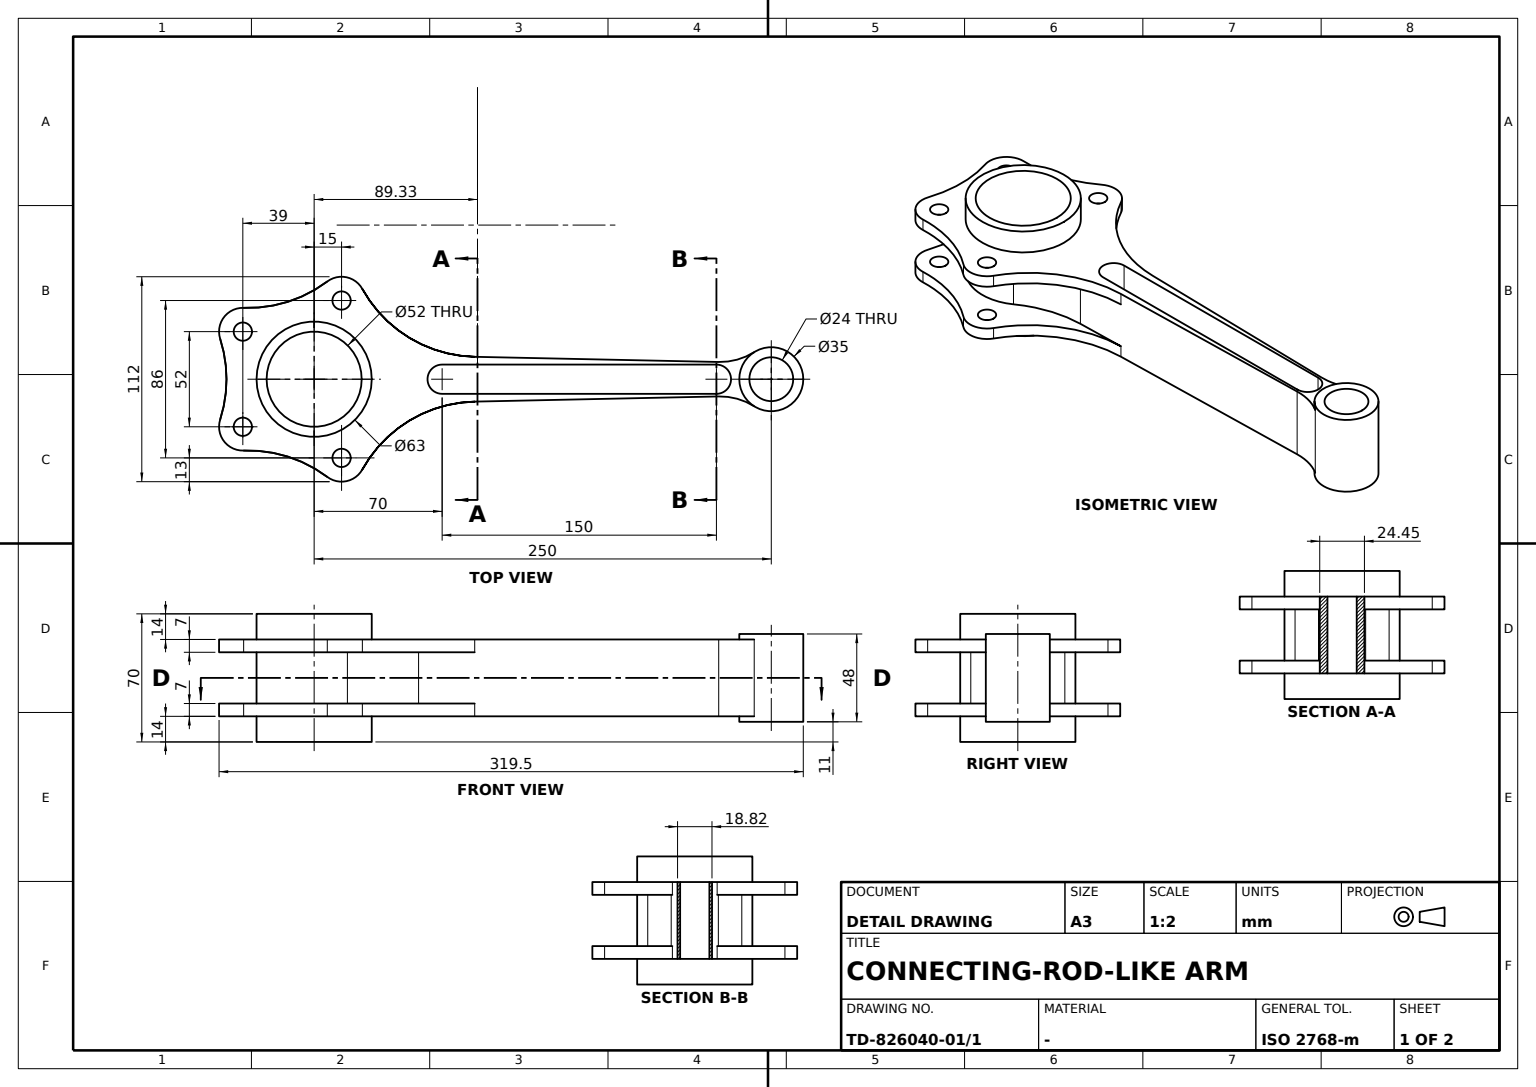
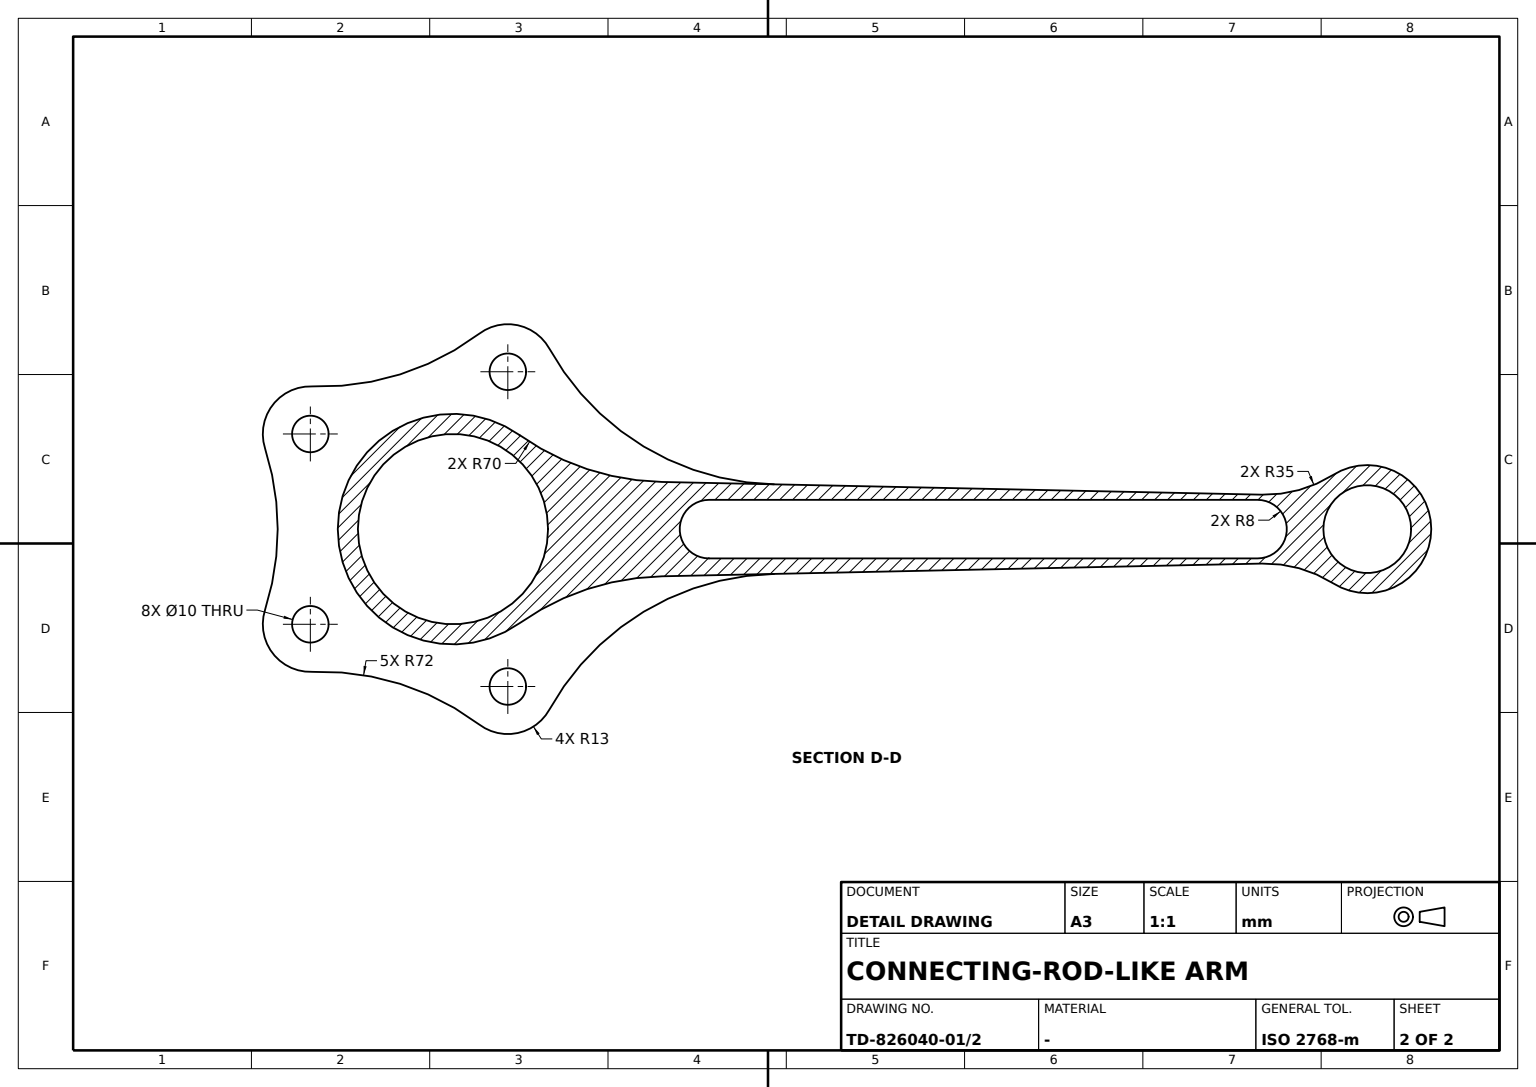
solid
v1 (7.189691,-53.392261,-14)
v2 (-38.551485,-38.992261,-14)
e1 v1 v2 CIRCLE(AX(P(-36.067402,-110.949396,-14),D(0,0,1),D(1,0,0)),72)
v3 (-38.551485,-38.992261,-21)
e2 v2 v3 LINE
v4 (7.189691,-53.392261,-21)
e3 v4 v3 CIRCLE(AX(P(-36.067402,-110.949396,-21),D(0,0,1),D(1,0,0)),72)
e4 v1 v4 LINE
face CYL(AX(P(-36.067402,-110.949396,17.5),D(0,0,1),D(1,0,0)),72) rev [e1 e2 -e3 -e4]
v5 (-38.551485,38.992261,-14)
v6 (7.189691,53.392261,-14)
e5 v5 v6 CIRCLE(AX(P(-36.067402,110.949396,-14),D(0,0,1),D(1,0,0)),72)
v7 (7.189691,53.392261,-21)
e6 v6 v7 LINE
v8 (-38.551485,38.992261,-21)
e7 v8 v7 CIRCLE(AX(P(-36.067402,110.949396,-21),D(0,0,1),D(1,0,0)),72)
e8 v5 v8 LINE
face CYL(AX(P(-36.067402,110.949396,17.5),D(0,0,1),D(1,0,0)),72) rev [e5 e6 -e7 -e8]
v9 (262,0,24)
e9 v9 v9 CIRCLE(AX(P(250,0,24),D(0,0,1),D(1,0,0)),12)
v10 (262,0,-24)
e10 v10 v10 CIRCLE(AX(P(250,0,-24),D(0,0,1),D(1,0,0)),12)
face CYL(AX(P(250,0,0),D(0,0,1),D(1,0,0)),12) rev [e9] [-e10]
v11 (31.5,0,-21)
e11 v11 v11 CIRCLE(AX(P(0,0,-21),D(0,0,1),D(1,0,0)),31.5)
v12 (31.5,0,-35)
e12 v12 v12 CIRCLE(AX(P(0,0,-35),D(0,0,1),D(1,0,0)),31.5)
face CYL(AX(P(0,0,0),D(0,0,1),D(1,0,0)),31.5) [-e11] [e12]
v13 (-51.376901,-22.023529,21)
v14 (-38.551485,-38.992261,21)
e13 v13 v14 CIRCLE(AX(P(-39,-26,21),D(0,0,1),D(1,0,0)),13)
v15 (-51.376901,-22.023529,14)
e14 v13 v15 LINE
v16 (-38.551485,-38.992261,14)
e15 v15 v16 CIRCLE(AX(P(-39,-26,14),D(0,0,1),D(1,0,0)),13)
e16 v14 v16 LINE
face CYL(AX(P(-39,-26,17.5),D(0,0,1),D(1,0,0)),13) [-e13 e14 e15 -e16]
v17 (57.116555,12.890905,-14)
v18 (57.116555,12.890905,14)
e17 v17 v18 LINE
v19 (87.808379,12.240359,14)
e18 v18 v19 LINE
v20 (87.808379,12.240359,21)
e19 v20 v19 LINE
v21 (221.248896,9.411947,21)
e20 v20 v21 LINE
v22 (221.248896,9.411947,-21)
e21 v22 v21 LINE
v23 (87.808379,12.240359,-21)
e22 v23 v22 LINE
v24 (87.808379,12.240359,-14)
e23 v24 v23 LINE
e24 v17 v24 LINE
face PLANE(AX(P(57.116555,12.890905,0),D(-0.02119129,-0.999775439,0),D(0.999775439,-0.02119129,0))) rev [e17 e18 -e19 e20 -e21 -e22 -e23 -e24]
v25 (-34,26,21)
e25 v25 v25 CIRCLE(AX(P(-39,26,21),D(0,0,1),D(1,0,0)),5)
v26 (-34,26,14)
e26 v26 v26 CIRCLE(AX(P(-39,26,14),D(0,0,1),D(1,0,0)),5)
face CYL(AX(P(-39,26,17.5),D(0,0,1),D(1,0,0)),5) rev [e25] [-e26]
v27 (26.368753,49.304876,21)
e27 v27 v20 CIRCLE(AX(P(89.334152,84.224191,21),D(0,0,1),D(1,0,0)),72)
v28 (26.368753,49.304876,14)
e28 v28 v19 CIRCLE(AX(P(89.334152,84.224191,14),D(0,0,1),D(1,0,0)),72)
e29 v27 v28 LINE
face CYL(AX(P(89.334152,84.224191,17.5),D(0,0,1),D(1,0,0)),72) rev [e27 e19 -e28 -e29]
v29 (20,43,-21)
e30 v29 v29 CIRCLE(AX(P(15,43,-21),D(0,0,1),D(1,0,0)),5)
v30 (240.66353,14.801363,-21)
e31 v22 v30 CIRCLE(AX(P(221.990591,44.404088,-21),D(0,0,1),D(1,0,0)),35)
v31 (240.66353,-14.801363,-21)
e32 v30 v31 CIRCLE(AX(P(250,0,-21),D(0,0,1),D(1,0,0)),17.5)
v32 (221.248896,-9.411947,-21)
e33 v31 v32 CIRCLE(AX(P(221.990591,-44.404088,-21),D(0,0,1),D(1,0,0)),35)
v33 (87.808379,-12.240359,-21)
e34 v33 v32 LINE
v34 (26.368753,-49.304876,-21)
e35 v33 v34 CIRCLE(AX(P(89.334152,-84.224191,-21),D(0,0,1),D(1,0,0)),72)
e36 v4 v34 CIRCLE(AX(P(15,-43,-21),D(0,0,1),D(1,0,0)),13)
v35 (-51.376901,-22.023529,-21)
e37 v35 v3 CIRCLE(AX(P(-39,-26,-21),D(0,0,1),D(1,0,0)),13)
v36 (-51.376901,22.023529,-21)
e38 v35 v36 CIRCLE(AX(P(-119.925892,0,-21),D(0,0,1),D(1,0,0)),72)
e39 v8 v36 CIRCLE(AX(P(-39,26,-21),D(0,0,1),D(1,0,0)),13)
v37 (26.368753,49.304876,-21)
e40 v37 v7 CIRCLE(AX(P(15,43,-21),D(0,0,1),D(1,0,0)),13)
e41 v37 v23 CIRCLE(AX(P(89.334152,84.224191,-21),D(0,0,1),D(1,0,0)),72)
v38 (-34,-26,-21)
e42 v38 v38 CIRCLE(AX(P(-39,-26,-21),D(0,0,1),D(1,0,0)),5)
v39 (20,-43,-21)
e43 v39 v39 CIRCLE(AX(P(15,-43,-21),D(0,0,1),D(1,0,0)),5)
v40 (-34,26,-21)
e44 v40 v40 CIRCLE(AX(P(-39,26,-21),D(0,0,1),D(1,0,0)),5)
v41 (70,8,-21)
v42 (220,8,-21)
e45 v41 v42 LINE
v43 (70,-8,-21)
e46 v41 v43 CIRCLE(AX(P(70,0,-21),D(0,0,1),D(1,0,0)),8)
v44 (220,-8,-21)
e47 v44 v43 LINE
e48 v44 v42 CIRCLE(AX(P(220,0,-21),D(0,0,1),D(1,0,0)),8)
face PLANE(AX(P(0,0,-21),D(0,0,1),D(1,0,0))) rev [e30] [e22 e31 e32 e33 -e34 e35 -e36 e3 -e37 e38 -e39 e7 -e40 e41] [e42] [e43] [e11] [e44] [-e45 e46 -e47 e48]
v45 (7.189691,-53.392261,14)
v46 (26.368753,-49.304876,14)
e49 v45 v46 CIRCLE(AX(P(15,-43,14),D(0,0,1),D(1,0,0)),13)
v47 (26.368753,-49.304876,21)
e50 v47 v46 LINE
v48 (7.189691,-53.392261,21)
e51 v48 v47 CIRCLE(AX(P(15,-43,21),D(0,0,1),D(1,0,0)),13)
e52 v48 v45 LINE
face CYL(AX(P(15,-43,17.5),D(0,0,1),D(1,0,0)),13) [e49 -e50 -e51 e52]
v49 (87.808379,-12.240359,-14)
e53 v33 v49 LINE
v50 (26.368753,-49.304876,-14)
e54 v49 v50 CIRCLE(AX(P(89.334152,-84.224191,-14),D(0,0,1),D(1,0,0)),72)
e55 v50 v34 LINE
face CYL(AX(P(89.334152,-84.224191,17.5),D(0,0,1),D(1,0,0)),72) rev [-e35 e53 e54 e55]
v51 (221.248896,-9.411947,21)
e56 v32 v51 LINE
v52 (87.808379,-12.240359,21)
e57 v52 v51 LINE
v53 (87.808379,-12.240359,14)
e58 v53 v52 LINE
v54 (57.116555,-12.890905,14)
e59 v54 v53 LINE
v55 (57.116555,-12.890905,-14)
e60 v55 v54 LINE
e61 v55 v49 LINE
face PLANE(AX(P(57.116555,-12.890905,0),D(0.02119129,-0.999775439,0),D(0.999775439,0.02119129,0))) [-e53 e34 e56 -e57 -e58 -e59 -e60 e61]
v56 (26.368753,49.304876,-14)
e62 v56 v6 CIRCLE(AX(P(15,43,-14),D(0,0,1),D(1,0,0)),13)
e63 v56 v37 LINE
face CYL(AX(P(15,43,17.5),D(0,0,1),D(1,0,0)),13) [e40 -e6 -e62 e63]
v57 (26,0,35)
e64 v57 v57 CIRCLE(AX(P(0,0,35),D(0,0,1),D(1,0,0)),26)
v58 (31.5,0,35)
e65 v58 v58 CIRCLE(AX(P(0,0,35),D(0,0,1),D(1,0,0)),31.5)
face PLANE(AX(P(0,0,35),D(0,0,1),D(1,0,0))) [-e64] [e65]
v59 (20,43,-14)
e66 v59 v59 CIRCLE(AX(P(15,43,-14),D(0,0,1),D(1,0,0)),5)
face CYL(AX(P(15,43,17.5),D(0,0,1),D(1,0,0)),5) rev [e66] [-e30]
v60 (-51.376901,22.023529,-14)
e67 v5 v60 CIRCLE(AX(P(-39,26,-14),D(0,0,1),D(1,0,0)),13)
e68 v60 v36 LINE
face CYL(AX(P(-39,26,17.5),D(0,0,1),D(1,0,0)),13) [-e67 e8 e39 -e68]
v61 (31.5,0,21)
e69 v61 v61 CIRCLE(AX(P(0,0,21),D(0,0,1),D(1,0,0)),31.5)
face CYL(AX(P(0,0,0),D(0,0,1),D(1,0,0)),31.5) [-e65] [e69]
v62 (18.18619,25.719885,14)
v63 (18.18619,-25.719885,14)
e70 v62 v63 CIRCLE(AX(P(0,0,14),D(0,0,1),D(1,0,0)),31.5)
v64 (18.18619,25.719885,-14)
e71 v64 v62 LINE
v65 (18.18619,-25.719885,-14)
e72 v64 v65 CIRCLE(AX(P(0,0,-14),D(0,0,1),D(1,0,0)),31.5)
e73 v65 v63 LINE
face CYL(AX(P(0,0,0),D(0,0,1),D(1,0,0)),31.5) [-e70 -e71 e72 e73]
v66 (267.5,0,-24)
e74 v66 v66 CIRCLE(AX(P(250,0,-24),D(0,0,1),D(1,0,0)),17.5)
face PLANE(AX(P(0,0,-24),D(0,0,1),D(1,0,0))) rev [-e74] [e10]
v67 (267.5,0,24)
e75 v67 v67 CIRCLE(AX(P(250,0,24),D(0,0,1),D(1,0,0)),17.5)
face PLANE(AX(P(0,0,24),D(0,0,1),D(1,0,0))) [-e9] [e75]
v68 (20,-43,21)
e76 v68 v68 CIRCLE(AX(P(15,-43,21),D(0,0,1),D(1,0,0)),5)
v69 (20,-43,14)
e77 v69 v69 CIRCLE(AX(P(15,-43,14),D(0,0,1),D(1,0,0)),5)
face CYL(AX(P(15,-43,17.5),D(0,0,1),D(1,0,0)),5) rev [e76] [-e77]
v70 (70,8,21)
v71 (220,8,21)
e78 v70 v71 LINE
e79 v70 v41 LINE
e80 v42 v71 LINE
face PLANE(AX(P(70,8,0),D(0,-1,0),D(1,0,0))) [-e78 e79 e45 e80]
v72 (-34,-26,14)
e81 v72 v72 CIRCLE(AX(P(-39,-26,14),D(0,0,1),D(1,0,0)),5)
v73 (20,43,14)
e82 v73 v73 CIRCLE(AX(P(15,43,14),D(0,0,1),D(1,0,0)),5)
e83 v62 v18 CIRCLE(AX(P(58.599946,82.875185,14),D(0,0,1),D(1,0,0)),70)
e84 v54 v63 CIRCLE(AX(P(58.599946,-82.875185,14),D(0,0,1),D(1,0,0)),70)
e85 v53 v46 CIRCLE(AX(P(89.334152,-84.224191,14),D(0,0,1),D(1,0,0)),72)
e86 v45 v16 CIRCLE(AX(P(-36.067402,-110.949396,14),D(0,0,1),D(1,0,0)),72)
v74 (-51.376901,22.023529,14)
e87 v15 v74 CIRCLE(AX(P(-119.925892,0,14),D(0,0,1),D(1,0,0)),72)
v75 (-38.551485,38.992261,14)
e88 v75 v74 CIRCLE(AX(P(-39,26,14),D(0,0,1),D(1,0,0)),13)
v76 (7.189691,53.392261,14)
e89 v75 v76 CIRCLE(AX(P(-36.067402,110.949396,14),D(0,0,1),D(1,0,0)),72)
e90 v28 v76 CIRCLE(AX(P(15,43,14),D(0,0,1),D(1,0,0)),13)
face PLANE(AX(P(0,0,14),D(0,0,1),D(1,0,0))) rev [e77] [e81] [e82] [e26] [-e18 -e83 e70 -e84 e59 e85 -e49 e86 -e15 e87 -e88 e89 -e90 e28]
v77 (220,-8,21)
e91 v77 v71 CIRCLE(AX(P(220,0,21),D(0,0,1),D(1,0,0)),8)
e92 v44 v77 LINE
face CYL(AX(P(220,0,0),D(0,0,1),D(1,0,0)),8) rev [e91 -e80 -e48 e92]
v78 (-34,-26,-14)
e93 v78 v78 CIRCLE(AX(P(-39,-26,-14),D(0,0,1),D(1,0,0)),5)
face CYL(AX(P(-39,-26,17.5),D(0,0,1),D(1,0,0)),5) rev [e93] [-e42]
e94 v1 v50 CIRCLE(AX(P(15,-43,-14),D(0,0,1),D(1,0,0)),13)
face CYL(AX(P(15,-43,17.5),D(0,0,1),D(1,0,0)),13) [e36 -e55 -e94 e4]
e95 v48 v14 CIRCLE(AX(P(-36.067402,-110.949396,21),D(0,0,1),D(1,0,0)),72)
face CYL(AX(P(-36.067402,-110.949396,17.5),D(0,0,1),D(1,0,0)),72) rev [e95 e16 -e86 -e52]
v79 (20,43,21)
e96 v79 v79 CIRCLE(AX(P(15,43,21),D(0,0,1),D(1,0,0)),5)
face CYL(AX(P(15,43,17.5),D(0,0,1),D(1,0,0)),5) rev [e96] [-e82]
v80 (-34,26,-14)
e97 v80 v80 CIRCLE(AX(P(-39,26,-14),D(0,0,1),D(1,0,0)),5)
e98 v64 v17 CIRCLE(AX(P(58.599946,82.875185,-14),D(0,0,1),D(1,0,0)),70)
e99 v56 v24 CIRCLE(AX(P(89.334152,84.224191,-14),D(0,0,1),D(1,0,0)),72)
v81 (-51.376901,-22.023529,-14)
e100 v81 v60 CIRCLE(AX(P(-119.925892,0,-14),D(0,0,1),D(1,0,0)),72)
e101 v81 v2 CIRCLE(AX(P(-39,-26,-14),D(0,0,1),D(1,0,0)),13)
e102 v55 v65 CIRCLE(AX(P(58.599946,-82.875185,-14),D(0,0,1),D(1,0,0)),70)
v82 (20,-43,-14)
e103 v82 v82 CIRCLE(AX(P(15,-43,-14),D(0,0,1),D(1,0,0)),5)
face PLANE(AX(P(0,0,-14),D(0,0,1),D(1,0,0))) [-e66] [-e93] [-e97] [-e72 e98 e24 -e99 e62 -e5 e67 -e100 e101 -e1 e94 -e54 -e61 e102] [-e103]
v83 (26,0,-35)
e104 v83 v83 CIRCLE(AX(P(0,0,-35),D(0,0,1),D(1,0,0)),26)
face CYL(AX(P(0,0,0),D(0,0,1),D(1,0,0)),26) rev [-e104] [e64]
v84 (70,-8,21)
e105 v70 v84 CIRCLE(AX(P(70,0,21),D(0,0,1),D(1,0,0)),8)
e106 v84 v43 LINE
face CYL(AX(P(70,0,0),D(0,0,1),D(1,0,0)),8) rev [-e79 e105 e106 -e46]
v85 (240.66353,-14.801363,21)
e107 v31 v85 LINE
v86 (240.66353,14.801363,21)
e108 v30 v86 LINE
e109 v86 v85 CIRCLE(AX(P(250,0,21),D(0,0,1),D(1,0,0)),17.5)
face CYL(AX(P(250,0,0),D(0,0,1),D(1,0,0)),17.5) [-e107 -e32 e108 e109] [e74] [-e75]
v87 (-51.376901,22.023529,21)
e110 v13 v87 CIRCLE(AX(P(-119.925892,0,21),D(0,0,1),D(1,0,0)),72)
e111 v87 v74 LINE
face CYL(AX(P(-119.925892,0,17.5),D(0,0,1),D(1,0,0)),72) rev [-e14 e110 e111 -e87]
face CYL(AX(P(58.599946,82.875185,0),D(0,0,1),D(1,0,0)),70) rev [-e17 -e98 e71 e83]
e112 v52 v47 CIRCLE(AX(P(89.334152,-84.224191,21),D(0,0,1),D(1,0,0)),72)
face CYL(AX(P(89.334152,-84.224191,17.5),D(0,0,1),D(1,0,0)),72) rev [-e85 e58 e112 e50]
face CYL(AX(P(-39,26,17.5),D(0,0,1),D(1,0,0)),5) rev [e97] [-e44]
face CYL(AX(P(58.599946,-82.875185,0),D(0,0,1),D(1,0,0)),70) rev [e60 e84 -e73 -e102]
v88 (-38.551485,38.992261,21)
v89 (7.189691,53.392261,21)
e113 v88 v89 CIRCLE(AX(P(-36.067402,110.949396,21),D(0,0,1),D(1,0,0)),72)
e114 v89 v76 LINE
e115 v88 v75 LINE
face CYL(AX(P(-36.067402,110.949396,17.5),D(0,0,1),D(1,0,0)),72) rev [e113 e114 -e89 -e115]
e116 v21 v86 CIRCLE(AX(P(221.990591,44.404088,21),D(0,0,1),D(1,0,0)),35)
face CYL(AX(P(221.990591,44.404088,0),D(0,0,1),D(1,0,0)),35) rev [e21 e116 -e108 -e31]
e117 v81 v35 LINE
face CYL(AX(P(-39,-26,17.5),D(0,0,1),D(1,0,0)),13) [-e101 e117 e37 -e2]
e118 v77 v84 LINE
face PLANE(AX(P(220,-8,0),D(0,1,0),D(-1,0,0))) [-e92 e47 -e106 -e118]
face CYL(AX(P(-119.925892,0,17.5),D(0,0,1),D(1,0,0)),72) rev [e68 -e38 -e117 e100]
face PLANE(AX(P(0,0,-35),D(0,0,1),D(1,0,0))) rev [e104] [-e12]
e119 v88 v87 CIRCLE(AX(P(-39,26,21),D(0,0,1),D(1,0,0)),13)
face CYL(AX(P(-39,26,17.5),D(0,0,1),D(1,0,0)),13) [e115 e88 -e111 -e119]
e120 v27 v89 CIRCLE(AX(P(15,43,21),D(0,0,1),D(1,0,0)),13)
face CYL(AX(P(15,43,17.5),D(0,0,1),D(1,0,0)),13) [-e114 -e120 e29 e90]
e121 v85 v51 CIRCLE(AX(P(221.990591,-44.404088,21),D(0,0,1),D(1,0,0)),35)
face CYL(AX(P(221.990591,-44.404088,0),D(0,0,1),D(1,0,0)),35) rev [e107 e121 -e56 -e33]
v90 (-34,-26,21)
e122 v90 v90 CIRCLE(AX(P(-39,-26,21),D(0,0,1),D(1,0,0)),5)
face PLANE(AX(P(0,0,21),D(0,0,1),D(1,0,0))) [-e122] [-e96] [-e76] [-e91 e118 -e105 e78] [-e25] [-e95 e51 -e112 e57 -e121 -e109 -e116 -e20 -e27 e120 -e113 e119 -e110 e13] [-e69]
face CYL(AX(P(15,-43,17.5),D(0,0,1),D(1,0,0)),5) rev [-e43] [e103]
face CYL(AX(P(-39,-26,17.5),D(0,0,1),D(1,0,0)),5) rev [e122] [-e81]
face CYL(AX(P(89.334152,84.224191,17.5),D(0,0,1),D(1,0,0)),72) rev [e99 e23 -e41 -e63]
